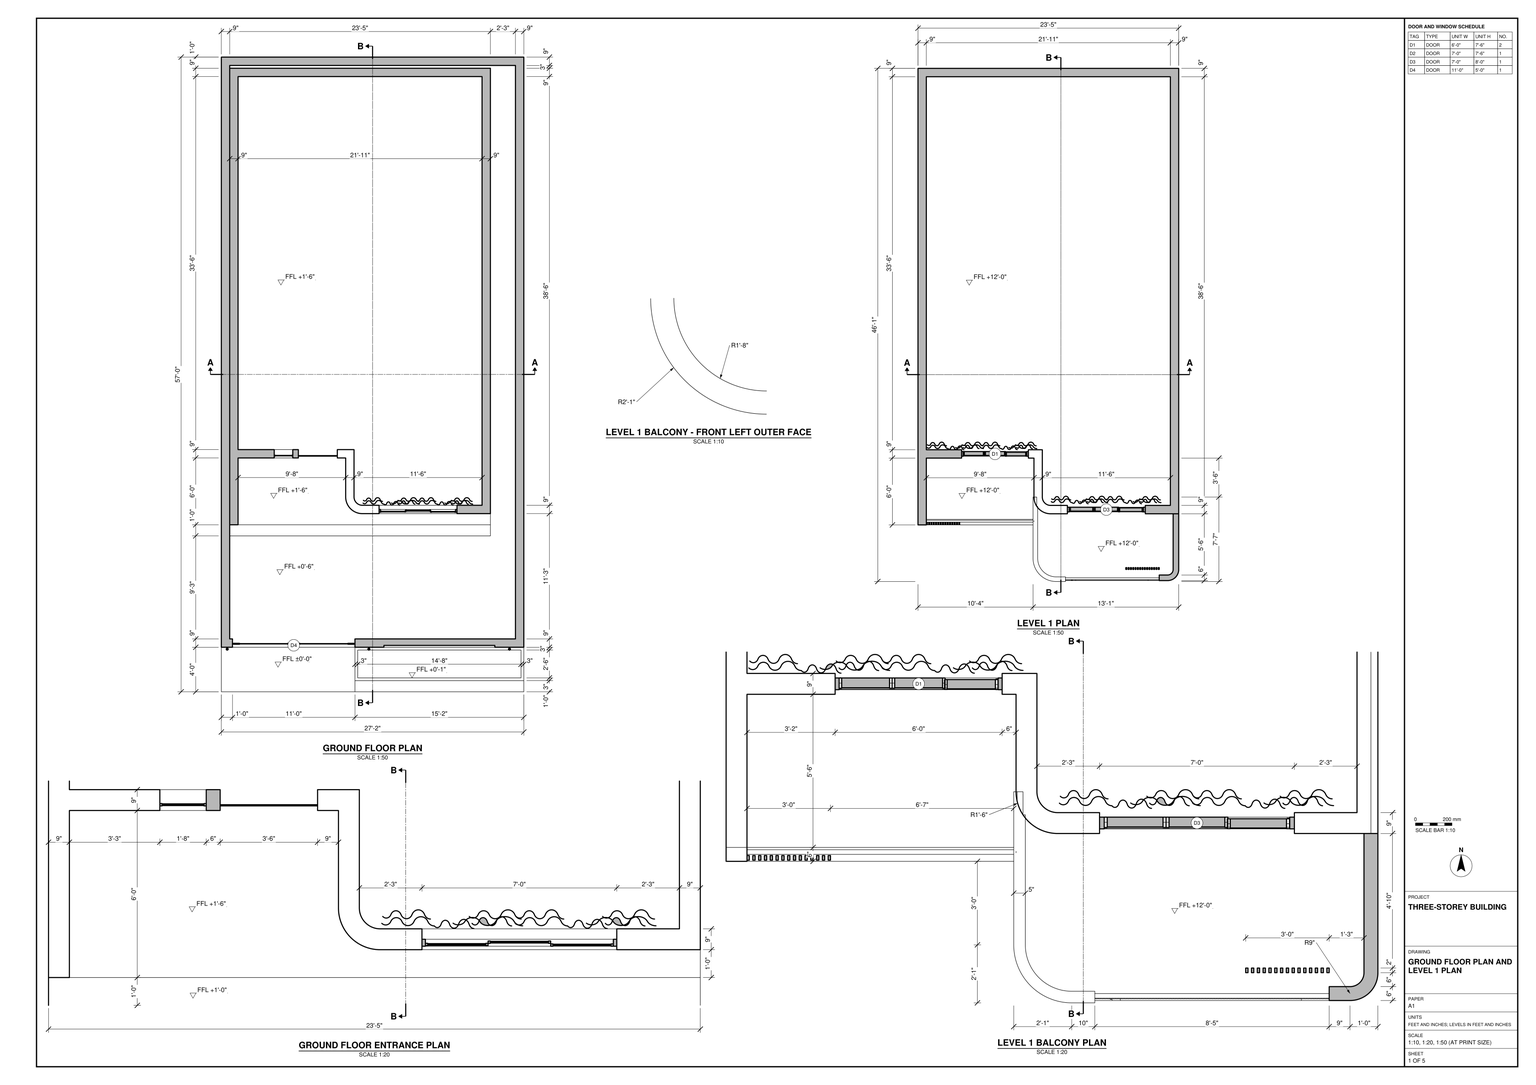
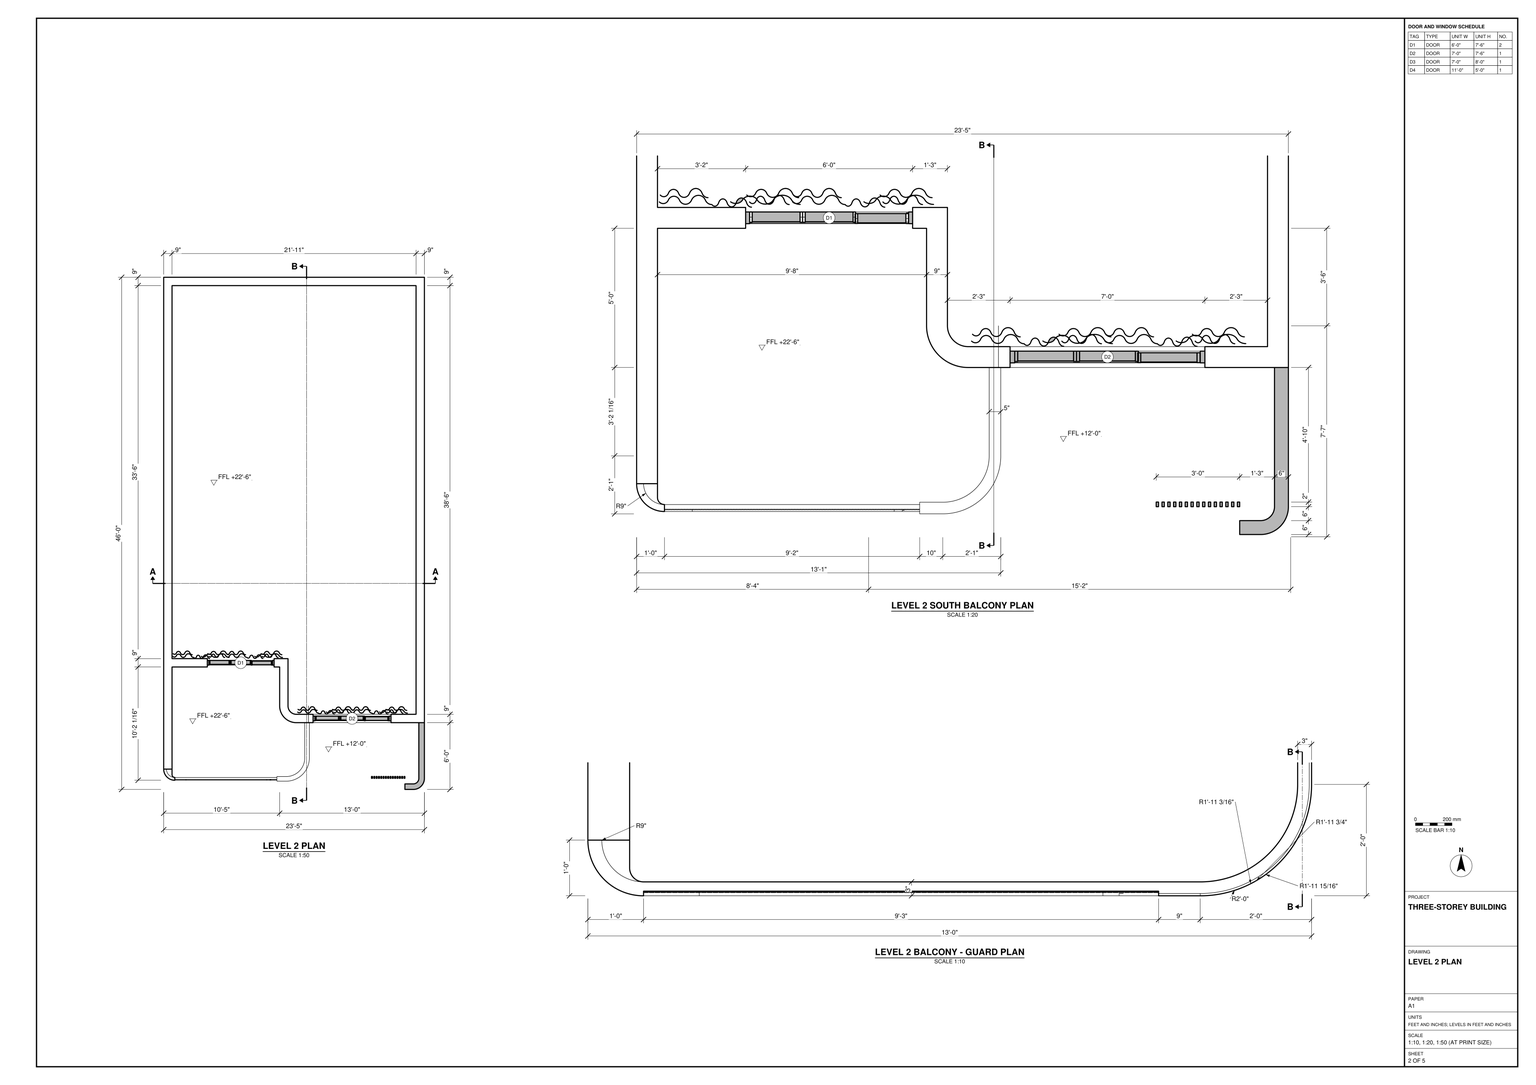
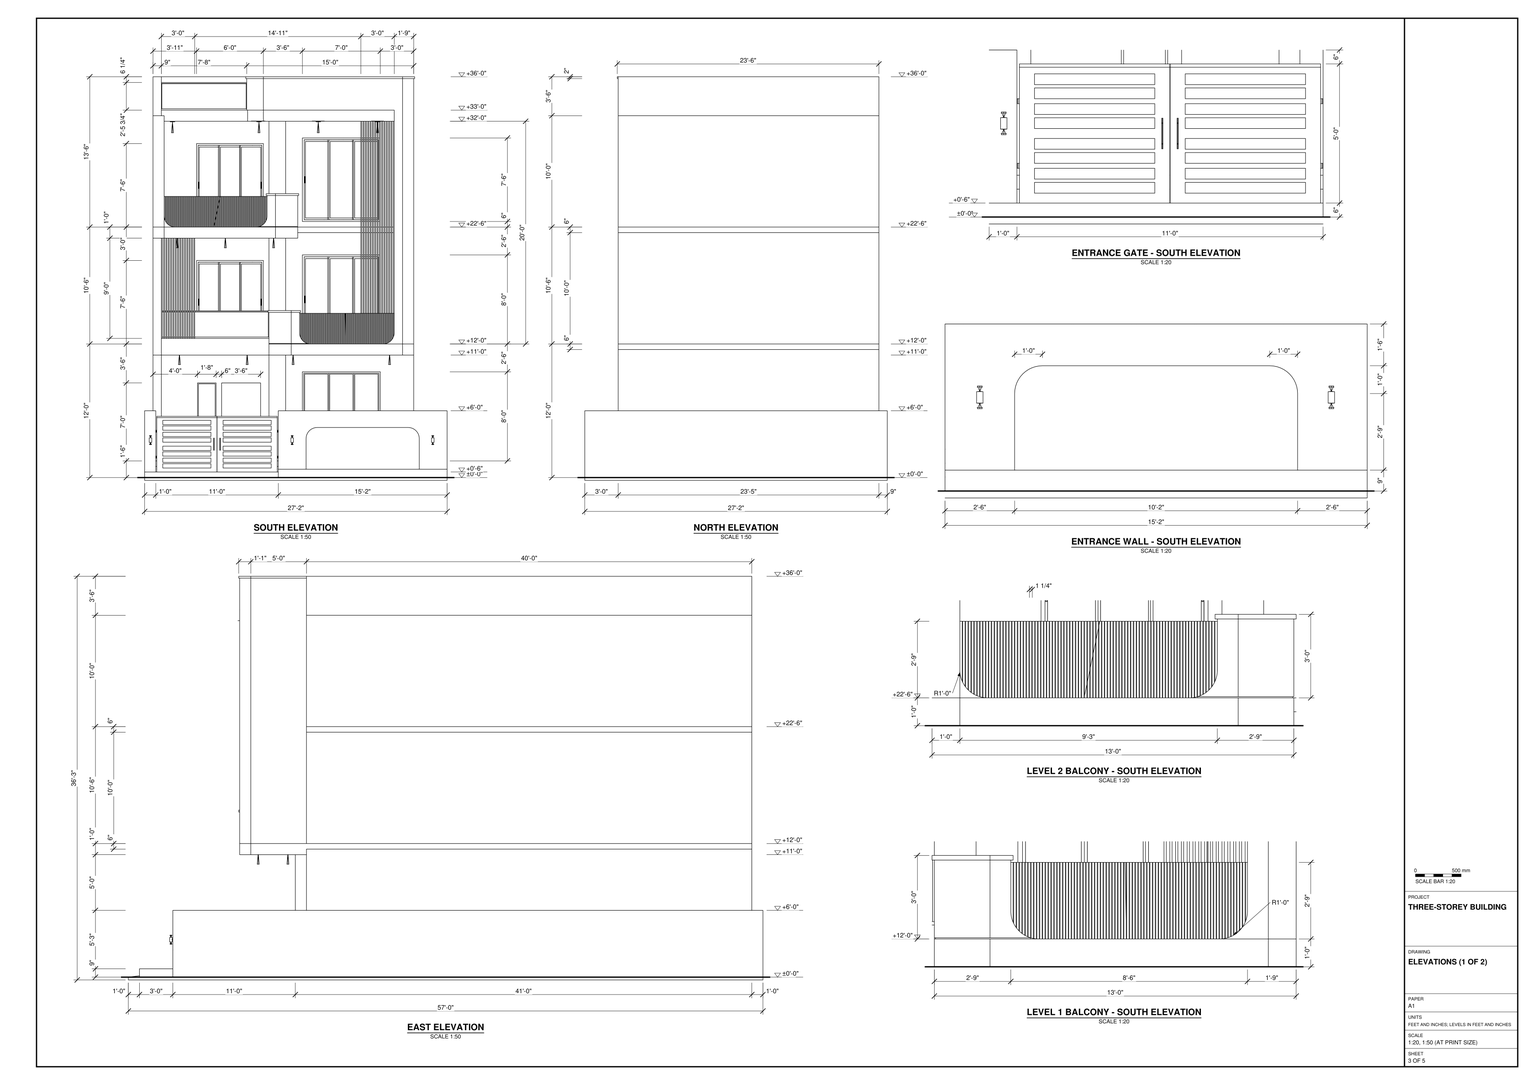
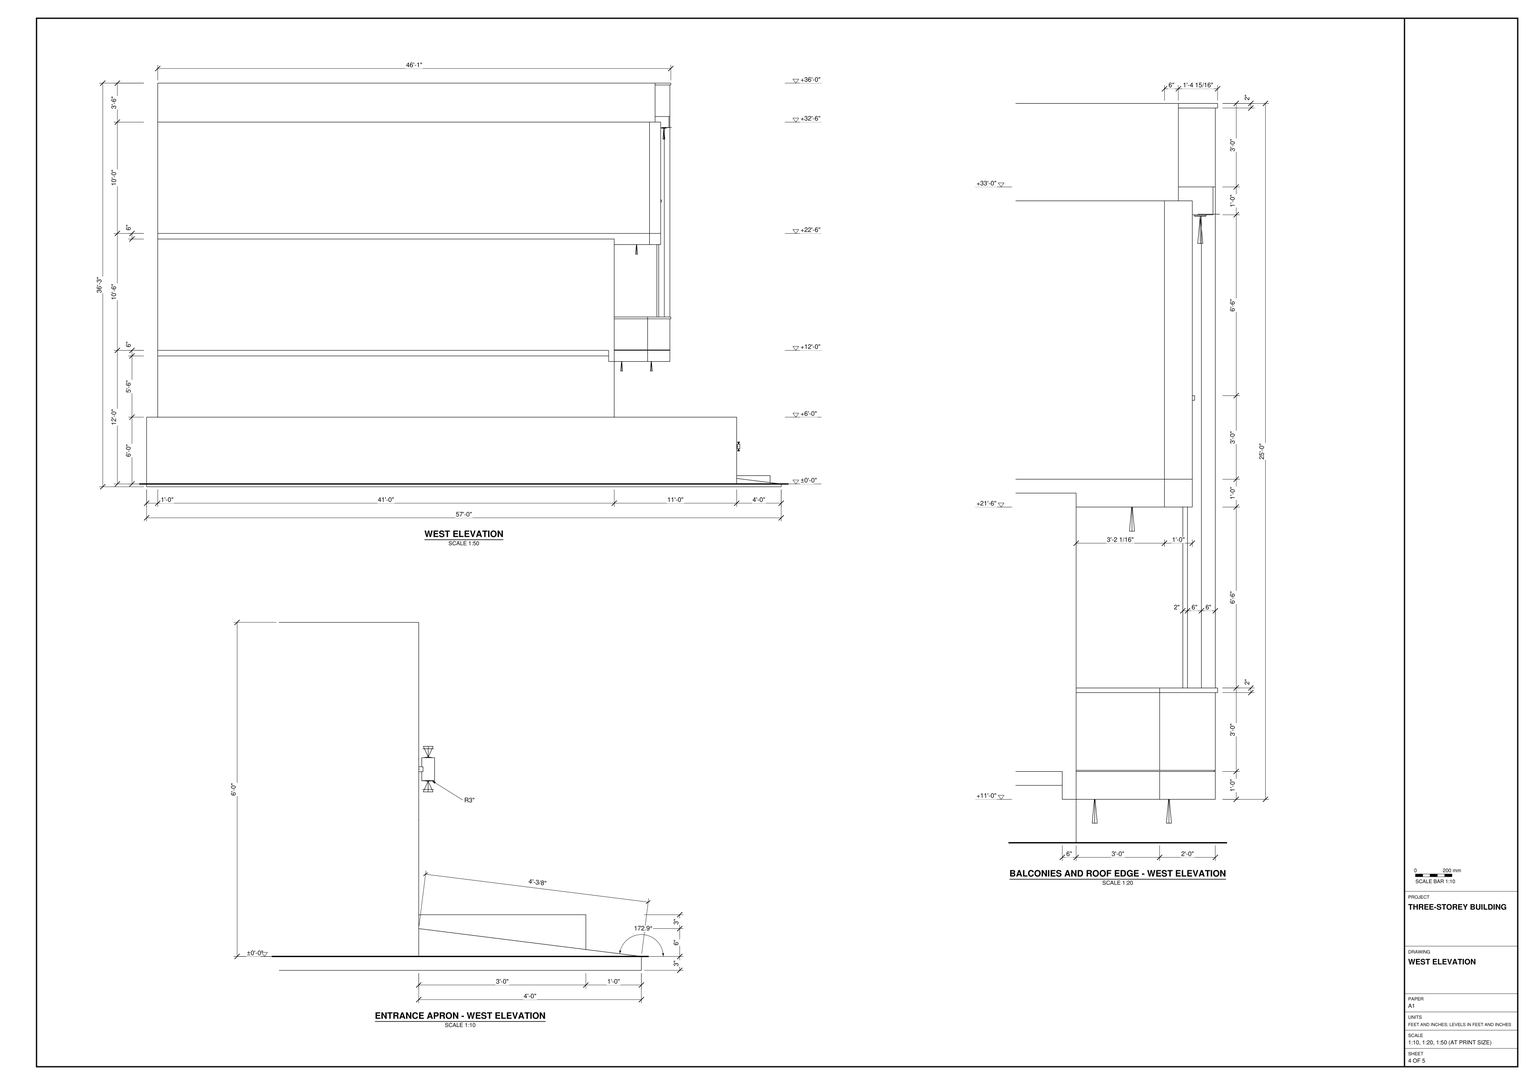
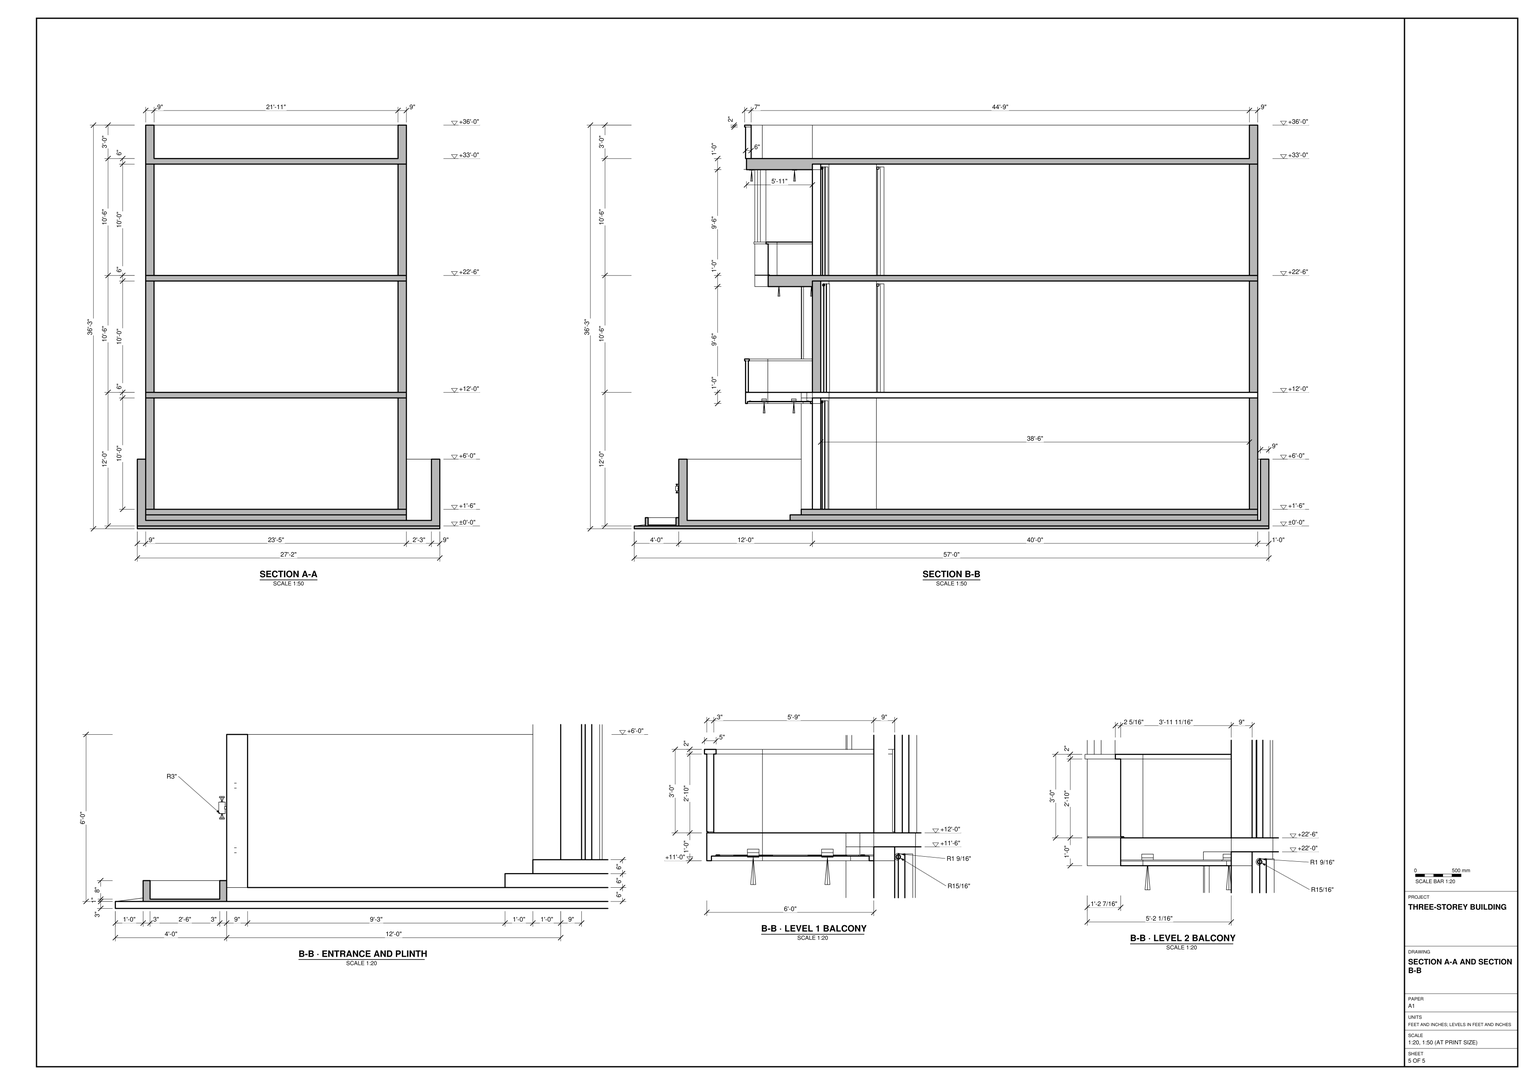
Build the three-storey building and its entrance court in SketchUp from task_files/diagram_01.pdf. Work in feet and inches. Including the court and boundary walls, the model must be 27'-2" wide, 57'-0" deep and 36'-3" high. Use ±0'-0" as the ground datum and set the upper floor levels at +12'-0" and +22'-6".

Start at the south boundary with the double-leaf gate on the left and the entrance wall on the right. Model the changes in height from the court up the shallow steps to the raised ground-floor entrance. Follow the plans for the 9" perimeter walls, the floor slabs and the offset front wall with its curved return. Fit the framed door units into the front openings, keeping the divisions shown in elevation. Leave the main floor areas open as drawn.

Project the level 1 balcony on the right and the level 2 balcony on the left as seen from the south. Use the enlarged details for their slab outlines, curved ends and guards. Distinguish the low balcony guards from the taller vertical screens behind them. Complete the flat roof and its projecting front edge. Keep shell elements such as walls, slabs and roof, and any furniture or joinery pieces, in separate groups or components; use components for repeated parts. Decor and loose items may be any suitable library components. Save one SketchUp model as output_files/three_storey_building_with_staggered_front_balconies.skp.

# SketchUp Ruby script. Lengths in inches.
U = 1.inch
M = Sketchup.active_model
def pt(a) = Geom::Point3d.new(a.map { |v| v * U })
def face(e, loops, mat)
  f = e.add_face(loops[0].map { |a| pt(a) })
  loops[1..].each { |l| e.add_face(l.map { |a| pt(a) }).erase! }
  f.material = f.back_material = mat if mat
  f
end
# faces: each face lists its corners as indices into pts; further lists are holes
def faces(e, pts, list, mat = nil) = list.each { |f| face(e, (f[0].is_a?(Array) ? f : [f]).map { |l| l.map { |i| pts[i] } }, mat) }
# xy, xz, yz: faces in a plane at the given z, y or x. An outline is a flat list of corners, or four numbers for a rectangle; further outlines are holes
def ring(l) = l.size == 4 ? [[l[0], l[1]], [l[2], l[1]], [l[2], l[3]], [l[0], l[3]]] : l.each_slice(2).to_a
def flat(e, list, mat, &to3) = list.each { |f| face(e, (f[0].is_a?(Array) ? f : [f]).map { |l| ring(l).map { |u, v| to3.(u, v) } }, mat) }
def xy(e, z, list, mat = nil) = flat(e, list, mat) { |x, y| [x, y, z] }
def xz(e, y, list, mat = nil) = flat(e, list, mat) { |x, z| [x, y, z] }
def yz(e, x, list, mat = nil) = flat(e, list, mat) { |y, z| [x, y, z] }
def lines(e, pts, list) = list.each { |a, b| e.add_line(pt(pts[a]), pt(pts[b])) }
# prism: a flat outline (further loops are holes) pulled along v
def prism(e, loops, v, mat = nil)
  f = face(e, loops, mat); d = Geom::Vector3d.new(v.map { |x| x * U })
  f.pushpull(f.normal.samedirection?(d) ? d.length : -d.length)
end
def box(e, o, s, mat = nil) = prism(e, [[o, [o[0] + s[0], o[1], o[2]], [o[0] + s[0], o[1] + s[1], o[2]], [o[0], o[1] + s[1], o[2]]]], [0, 0, s[2]], mat)
def at(x, y, z, deg = 0) = Geom::Transformation.translation(pt([x, y, z])) * Geom::Transformation.rotation(ORIGIN, Z_AXIS, deg.degrees)
def axes(o, x, y, z) = Geom::Transformation.new([*x, 0, *y, 0, *z, 0, *pt(o).to_a, 1])
def part(name) = M.definitions.add(name)
# library, detail: a bought-in or finely detailed component or shape, given as its bounding box
def library(name, o, s) = part(name).tap { |d| box(d.entities, o, s) }
def detail(e, o, s) = box(e.add_group.entities, o, s)
def put(e, d, t, mat = nil) = e.add_instance(d, t).tap { |i| i.material = mat if mat }
def group(e, t, mat = nil) = e.add_group.tap { |g| g.transformation = t; g.material = mat if mat }.entities
root = M.entities
M.materials.add("1422 AP 8231 MUTED GREY").color = [95, 93, 94]
M.materials.add("1423 AP 8230 BENTONITE").color = [77, 75, 77]
M.materials.add("1427 AP 686 ARMOUR-N").color = [184, 186, 189]
M.materials.add("[Concrete Block 8x8 Gray]").color = [94, 94, 94]
M.materials.add("[Granite Tile]").color = [155, 148, 143]
M.materials.add("[Granite Tile]1").color = [155, 148, 143]
M.materials.add("[Translucent Glass Blue]").color = [185, 200, 227]
M.materials.add("[Wood Cherry Original]").color = [100, 65, 42]
M.materials.add("[Wood Veneer 01]").color = [99, 65, 43]
c1 = library("Group\#8",[0,-72,0],[281,492,120])
c2 = library("Group\#2",[0,-110.08,0],[281,530.08,120])
c3 = library("Group\#14",[0,-72,-12],[281,492,132])
c4 = library("Group\#13",[-25,-1,0],[182,91,288])
c5 = library("Group\#7",[-9,-81,-16.28],[281,552,58.03])
c6 = library("Group\#12",[-9,-71.08,-16.4],[281,542.08,22.4])
c7 = library("Group\#9",[-1,-1,0],[157,81.05,120])
c8 = part("Group188\#1")
box(c8.entities,[-18,-57,0],[1,114,2])
c9 = part("Group189\#1")
box(c9.entities,[-15.5,-57,0],[1,114,2])
c10 = part("Group190\#1")
box(c10.entities,[-13,-57,0],[1,114,2])
c11 = part("Group191\#1")
box(c11.entities,[-10.5,-57,0],[1,114,2])
c12 = part("Group192\#1")
box(c12.entities,[-8,-57,0],[1,114,2])
c13 = part("Group193\#1")
box(c13.entities,[-5.5,-57,0],[1,114,2])
c14 = part("Group194\#1")
box(c14.entities,[-3,-57,0],[1,114,2])
c15 = part("Group195\#1")
box(c15.entities,[-0.5,-57,0],[1,114,2])
c16 = part("Group196\#1")
box(c16.entities,[2,-57,0],[1,114,2])
c17 = part("Group197\#1")
box(c17.entities,[4.5,-57,0],[1,114,2])
c18 = part("Group198\#1")
box(c18.entities,[7,-57,0],[1,114,2])
c19 = part("Group199\#1")
box(c19.entities,[9.5,-57,0],[1,114,2])
c20 = part("Group200\#1")
box(c20.entities,[12,-57,0],[1,114,2])
c21 = part("Group201\#1")
box(c21.entities,[14.5,-57,0],[1,114,2])
c22 = part("Group202\#1")
box(c22.entities,[17,-57,0],[1,114,2])
c23 = part("Group186\#1")
put(c23.entities,c8,at(0,0,0))
put(c23.entities,c9,at(0,0,0))
put(c23.entities,c10,at(0,0,0))
put(c23.entities,c11,at(0,0,0))
put(c23.entities,c12,at(0,0,0))
put(c23.entities,c13,at(0,0,0))
put(c23.entities,c14,at(0,0,0))
put(c23.entities,c15,at(0,0,0))
put(c23.entities,c16,at(0,0,0))
put(c23.entities,c17,at(0,0,0))
put(c23.entities,c18,at(0,0,0))
put(c23.entities,c19,at(0,0,0))
put(c23.entities,c20,at(0,0,0))
put(c23.entities,c21,at(0,0,0))
put(c23.entities,c22,at(0,0,0))
c24 = part("Group\#19")
put(c24.entities,c23,axes([18,0,57],[1,0,0],[0,0,1],[0,-1,0]))
c25 = library("Group\#15",[-9,-82.92,-18.4],[281,553.92,60.4])
c26 = library("Gate",[-1,-3.25,0],[122,4.25,84])
c27 = library("WALL LIGHT 69\#1",[4.19,4.05,-8.39],[4.61,5.7,16.35])
g1 = group(root,at(9,252,0))
g2 = group(g1,at(0,-133,-12))
box(g2,[9,37.5,378],[93,11,12],"1423 AP 8230 BENTONITE")
put(g2,c1,at(0,133,12),"1427 AP 686 ARMOUR-N")
put(g2,c2,at(0,133,264),"1427 AP 686 ARMOUR-N")
put(g2,c3,at(0,133,138),"1423 AP 8230 BENTONITE")
g3 = group(g2,at(0,73,6),"[Granite Tile]")
box(g3,[0,-24,-6],[281,504,6])
g4 = group(g2,at(0,73,12),"[Granite Tile]")
box(g4,[0,-12,-6],[281,492,6])
put(g2,c4,at(125,1,138),"1427 AP 686 ARMOUR-N")
put(g2,c5,at(9,82,132))
put(g2,c6,at(9,82,258))
put(g2,c7,axes([156,10.92,264],[-1,0,0],[0,1,0],[0,0,1]),"1427 AP 686 ARMOUR-N")
put(g2,c24,axes([9,63.5,144],[1,0,0],[0,1,0],[0,0,0.94737]),"[Wood Cherry Original]")
put(g2,c24,axes([224,15,138],[1,0,0],[0,1,0],[0,0,2.10526]),"[Wood Cherry Original]")
put(g2,c25,at(9,82,384))
g5 = group(g2,at(37.55,69,390),"[Wood Veneer 01]")
xy(g5,0,[[-28.55,0,63.45,2]])
xy(g5,1.25,[[-27.96,0.75,62.85,1.25]])
xy(g5,1.5,[[[-28.55,0,63.45,2],[-27.96,0.75,62.85,1.25]]])
xy(g5,28.5,[[-28.55,0.2,63.45,0.23],[-28.55,0.23,63.45,0.25],[[-28.55,0.25,63.45,1.75],[-27.96,0.75,62.85,1.25]],[-28.55,1.75,63.45,1.77],[-28.55,1.77,63.45,1.8]])
xy(g5,28.75,[[-27.96,0.75,62.85,1.25]])
xy(g5,29.74,[[-28.55,0.84,63.45,0.9],[-28.55,1.1,63.45,1.16]])
xy(g5,29.75,[[-28.55,0.95,63.45,1],[-28.55,1,63.45,1.05]])
xz(g5,0,[[-28.55,0,63.45,1.5],[-28.55,28.7,63.45,28.73],[-28.55,28.73,63.45,28.75],[-28.55,28.75,63.45,28.8]])
xz(g5,0.01,[[-28.55,28.85,63.45,28.91]])
xz(g5,0.75,[[-27.96,1.25,62.85,1.5],[-27.96,28.5,62.85,28.75]])
xz(g5,1.25,[[-27.96,1.25,62.85,1.5],[-27.96,28.5,62.85,28.75]])
xz(g5,1.99,[[-28.55,28.85,63.45,28.91]])
xz(g5,2,[[-28.55,0,63.45,1.5],[-28.55,28.7,63.45,28.73],[-28.55,28.73,63.45,28.75],[-28.55,28.75,63.45,28.8]])
yz(g5,-28.55,[[0,0,2,1.5],[0.2,28.5,0.18,28.51,0.15,28.52,0.11,28.54,0.09,28.56,0.07,28.57,0.06,28.59,0.04,28.61,0.02,28.65,0.01,28.68,0,28.7,0,28.8,0.01,28.85,0.01,28.91,0.03,29.01,0.09,29.16,0.11,29.2,0.13,29.25,0.16,29.29,0.19,29.34,0.22,29.38,0.26,29.42,0.29,29.46,0.33,29.49,0.37,29.53,0.41,29.56,0.46,29.59,0.5,29.62,0.55,29.64,0.59,29.66,0.74,29.72,0.84,29.74,0.9,29.74,0.95,29.75,1.05,29.75,1.1,29.74,1.16,29.74,1.26,29.72,1.41,29.66,1.45,29.64,1.5,29.62,1.54,29.59,1.59,29.56,1.63,29.53,1.67,29.49,1.71,29.46,1.74,29.42,1.78,29.38,1.81,29.34,1.84,29.29,1.87,29.25,1.89,29.2,1.91,29.16,1.97,29.01,1.99,28.91,1.99,28.85,2,28.8,2,28.7,1.99,28.68,1.98,28.65,1.96,28.61,1.94,28.59,1.93,28.57,1.91,28.56,1.89,28.54,1.85,28.52,1.82,28.51,1.8,28.5]])
yz(g5,-27.96,[[0.75,1.25,1.25,1.5],[0.75,28.5,1.25,28.75]])
yz(g5,62.85,[[0.75,1.25,1.25,1.5],[0.75,28.5,1.25,28.75]])
yz(g5,63.45,[[0,0,2,1.5],[0.2,28.5,1.8,28.5,1.82,28.51,1.85,28.52,1.89,28.54,1.91,28.56,1.93,28.57,1.94,28.59,1.96,28.61,1.98,28.65,1.99,28.68,2,28.7,2,28.8,1.99,28.85,1.99,28.91,1.97,29.01,1.91,29.16,1.89,29.2,1.87,29.25,1.84,29.29,1.81,29.34,1.78,29.38,1.74,29.42,1.71,29.46,1.67,29.49,1.63,29.53,1.59,29.56,1.54,29.59,1.5,29.62,1.45,29.64,1.41,29.66,1.26,29.72,1.16,29.74,1.1,29.74,1.05,29.75,0.95,29.75,0.9,29.74,0.84,29.74,0.74,29.72,0.59,29.66,0.55,29.64,0.5,29.62,0.46,29.59,0.41,29.56,0.37,29.53,0.33,29.49,0.29,29.46,0.26,29.42,0.22,29.38,0.19,29.34,0.16,29.29,0.13,29.25,0.11,29.2,0.09,29.16,0.03,29.01,0.01,28.91,0.01,28.85,0,28.8,0,28.7,0.01,28.68,0.02,28.65,0.04,28.61,0.06,28.59,0.07,28.57,0.09,28.56,0.11,28.54,0.15,28.52,0.18,28.51]])
p = [[-28.55,0.13,28.53],[-28.55,0.15,28.52],[63.45,0.15,28.52],[63.45,0.13,28.53],[-28.55,0.11,28.54],[63.45,0.11,28.54],
  [-28.55,0.09,28.56],[63.45,0.09,28.56],[-28.55,0.18,28.51],[-28.55,0.2,28.5],[63.45,0.2,28.5],[63.45,0.18,28.51],
  [-28.55,1.85,28.52],[-28.55,1.87,28.53],[63.45,1.87,28.53],[63.45,1.85,28.52],[-28.55,1.82,28.51],[63.45,1.82,28.51],
  [-28.55,1.8,28.5],[63.45,1.8,28.5],[-28.55,1.89,28.54],[-28.55,1.91,28.56],[63.45,1.91,28.56],[63.45,1.89,28.54],
  [-28.55,0.04,28.61],[-28.55,0.06,28.59],[63.45,0.06,28.59],[63.45,0.04,28.61],[-28.55,0.03,28.63],[63.45,0.03,28.63],
  [-28.55,0.02,28.65],[63.45,0.02,28.65],[-28.55,0.07,28.57],[63.45,0.07,28.57],[-28.55,1.94,28.59],[-28.55,1.96,28.61],
  [63.45,1.96,28.61],[63.45,1.94,28.59],[-28.55,1.93,28.57],[63.45,1.93,28.57],[-28.55,1.97,28.63],[-28.55,1.98,28.65],
  [63.45,1.98,28.65],[63.45,1.97,28.63],[-28.55,0.01,28.68],[63.45,0.01,28.68],[-28.55,0,28.7],[63.45,0,28.7],
  [-28.55,1.99,28.68],[-28.55,2,28.7],[63.45,2,28.7],[63.45,1.99,28.68],[-28.55,0.01,28.85],[-28.55,0,28.8],
  [63.45,0,28.8],[63.45,0.01,28.85],[-28.55,2,28.8],[-28.55,1.99,28.85],[63.45,1.99,28.85],[63.45,2,28.8],
  [-28.55,0.02,28.96],[-28.55,0.01,28.91],[63.45,0.01,28.91],[63.45,0.02,28.96],[-28.55,1.99,28.91],[-28.55,1.98,28.96],
  [63.45,1.98,28.96],[63.45,1.99,28.91],[-28.55,0.03,29.01],[63.45,0.03,29.01],[-28.55,0.05,29.06],[63.45,0.05,29.06],
  [-28.55,1.97,29.01],[-28.55,1.95,29.06],[63.45,1.95,29.06],[63.45,1.97,29.01],[-28.55,0.07,29.11],[63.45,0.07,29.11],
  [-28.55,0.09,29.16],[63.45,0.09,29.16],[-28.55,1.93,29.11],[-28.55,1.91,29.16],[63.45,1.91,29.16],[63.45,1.93,29.11],
  [-28.55,0.11,29.2],[63.45,0.11,29.2],[-28.55,0.13,29.25],[63.45,0.13,29.25],[-28.55,1.89,29.2],[-28.55,1.87,29.25],
  [63.45,1.87,29.25],[63.45,1.89,29.2],[-28.55,0.16,29.29],[63.45,0.16,29.29],[-28.55,0.19,29.34],[63.45,0.19,29.34],
  [-28.55,0.22,29.38],[63.45,0.22,29.38],[-28.55,1.81,29.34],[-28.55,1.78,29.38],[63.45,1.78,29.38],[63.45,1.81,29.34],
  [-28.55,1.84,29.29],[63.45,1.84,29.29],[-28.55,0.26,29.42],[63.45,0.26,29.42],[-28.55,0.29,29.46],[63.45,0.29,29.46],
  [-28.55,1.74,29.42],[-28.55,1.71,29.46],[63.45,1.71,29.46],[63.45,1.74,29.42],[-28.55,0.33,29.49],[63.45,0.33,29.49],
  [-28.55,0.37,29.53],[63.45,0.37,29.53],[-28.55,0.41,29.56],[63.45,0.41,29.56],[-28.55,1.63,29.53],[-28.55,1.59,29.56],
  [63.45,1.59,29.56],[63.45,1.63,29.53],[-28.55,1.67,29.49],[63.45,1.67,29.49],[-28.55,0.46,29.59],[63.45,0.46,29.59],
  [-28.55,0.5,29.62],[63.45,0.5,29.62],[-28.55,0.55,29.64],[63.45,0.55,29.64],[-28.55,0.59,29.66],[63.45,0.59,29.66],
  [-28.55,1.45,29.64],[-28.55,1.41,29.66],[63.45,1.41,29.66],[63.45,1.45,29.64],[-28.55,1.5,29.62],[63.45,1.5,29.62],
  [-28.55,1.54,29.59],[63.45,1.54,29.59],[-28.55,0.64,29.68],[63.45,0.64,29.68],[-28.55,0.69,29.7],[63.45,0.69,29.7],
  [-28.55,0.74,29.72],[63.45,0.74,29.72],[-28.55,0.79,29.73],[63.45,0.79,29.73],[-28.55,0.84,29.74],[63.45,0.84,29.74],
  [-28.55,0.95,29.75],[-28.55,0.9,29.74],[63.45,0.9,29.74],[63.45,0.95,29.75],[-28.55,1.1,29.74],[-28.55,1.05,29.75],
  [63.45,1.05,29.75],[63.45,1.1,29.74],[-28.55,1.21,29.73],[-28.55,1.16,29.74],[63.45,1.16,29.74],[63.45,1.21,29.73],
  [-28.55,1.26,29.72],[63.45,1.26,29.72],[-28.55,1.31,29.7],[63.45,1.31,29.7],[-28.55,1.36,29.68],[63.45,1.36,29.68]]
faces(g5,p,[[0,1,2,3],[4,0,3,5],[6,4,5,7],[8,9,10,11],[1,8,11,2],[12,13,14,15],[16,12,15,17],[18,16,17,19],
  [20,21,22,23],[13,20,23,14],[24,25,26,27],[28,24,27,29],[30,28,29,31],[32,6,7,33],[25,32,33,26],[34,35,36,37],
  [38,34,37,39],[21,38,39,22],[40,41,42,43],[35,40,43,36],[44,30,31,45],[46,44,45,47],[48,49,50,51],[41,48,51,42],
  [52,53,54,55],[56,57,58,59],[60,61,62,63],[64,65,66,67],[68,60,63,69],[70,68,69,71],[72,73,74,75],[65,72,75,66],
  [76,70,71,77],[78,76,77,79],[80,81,82,83],[73,80,83,74],[84,78,79,85],[86,84,85,87],[88,89,90,91],[81,88,91,82],
  [92,86,87,93],[94,92,93,95],[96,94,95,97],[98,99,100,101],[102,98,101,103],[89,102,103,90],[104,96,97,105],[106,104,105,107],
  [108,109,110,111],[99,108,111,100],[112,106,107,113],[114,112,113,115],[116,114,115,117],[118,119,120,121],[122,118,121,123],[109,122,123,110],
  [124,116,117,125],[126,124,125,127],[128,126,127,129],[130,128,129,131],[132,133,134,135],[136,132,135,137],[138,136,137,139],[119,138,139,120],
  [140,130,131,141],[142,140,141,143],[144,142,143,145],[146,144,145,147],[148,146,147,149],[150,151,152,153],[154,155,156,157],[158,159,160,161],
  [162,158,161,163],[164,162,163,165],[166,164,165,167],[133,166,167,134]])
g6 = group(g5,at(0.59,0.75,1.25),"[Translucent Glass Blue]")
box(g6,[-28.55,0,0],[90.81,0.5,27.5])
g7 = group(g2,at(0,49,0),"1427 AP 686 ARMOUR-N")
xy(g7,-6,[[-9,-120,-9,516,317,516,317,-120,287,-120,287,-118,165,-118,165,-120],[165,-120,287,-118]])
xy(g7,0,[[3,-120,135,-120,135,-111,308,-111,308,507,0,507,0,-111,3,-111]],"[Granite Tile]")
xy(g7,48,[[177,-120,275,-118]])
xy(g7,66,[[-9,-120,3,-120,3,-111,0,-111,0,507,308,507,308,-111,135,-111,135,-120,317,-120,317,516,-9,516]])
xz(g7,-120,[[-9,-6,165,-6,165,36,165.1,37.57,165.41,39.11,165.91,40.59,166.61,42,167.48,43.31,168.51,44.49,169.69,45.52,171,46.39,172.41,47.09,173.89,47.59,175.43,47.9,177,48,275,48,276.57,47.9,278.11,47.59,279.59,47.09,281,46.39,282.31,45.52,283.49,44.49,284.52,43.31,285.39,42,286.09,40.59,286.59,39.11,286.9,37.57,287,36,287,-6,317,-6,317,66,135,66,135,0,3,0,3,66,-9,66]])
xz(g7,-118,[[165,-6,287,-6,287,36,286.9,37.57,286.59,39.11,286.09,40.59,285.39,42,284.52,43.31,283.49,44.49,282.31,45.52,281,46.39,279.59,47.09,278.11,47.59,276.57,47.9,275,48,177,48,175.43,47.9,173.89,47.59,172.41,47.09,171,46.39,169.69,45.52,168.51,44.49,167.48,43.31,166.61,42,165.91,40.59,165.41,39.11,165.1,37.57,165,36]],"1422 AP 8231 MUTED GREY")
xz(g7,-111,[[0,0,3,66],[135,0,308,66]])
xz(g7,507,[[0,0,308,66]])
xz(g7,516,[[-9,-6,317,66]])
yz(g7,-9,[[-120,-6,516,66]])
yz(g7,0,[[-111,0,507,66]])
yz(g7,3,[[-120,0,-111,66]])
yz(g7,135,[[-120,0,-111,66]])
yz(g7,165,[[-120,-6,-118,36]])
yz(g7,287,[[-120,-6,-118,36]])
yz(g7,308,[[-111,0,507,66]])
yz(g7,317,[[-120,-6,516,66]])
p = [[165.1,-120,37.57],[165,-120,36],[165,-118,36],[165.1,-118,37.57],[287,-120,36],[286.9,-120,37.57],
  [286.9,-118,37.57],[287,-118,36],[165.41,-120,39.11],[165.41,-118,39.11],[286.59,-120,39.11],[286.59,-118,39.11],
  [165.91,-120,40.59],[165.91,-118,40.59],[286.09,-120,40.59],[286.09,-118,40.59],[166.61,-120,42],[166.61,-118,42],
  [285.39,-120,42],[285.39,-118,42],[167.48,-120,43.31],[167.48,-118,43.31],[284.52,-120,43.31],[284.52,-118,43.31],
  [168.51,-120,44.49],[168.51,-118,44.49],[283.49,-120,44.49],[283.49,-118,44.49],[169.69,-120,45.52],[169.69,-118,45.52],
  [282.31,-120,45.52],[282.31,-118,45.52],[171,-120,46.39],[171,-118,46.39],[281,-120,46.39],[281,-118,46.39],
  [172.41,-120,47.09],[172.41,-118,47.09],[279.59,-120,47.09],[279.59,-118,47.09],[173.89,-120,47.59],[173.89,-118,47.59],
  [278.11,-120,47.59],[278.11,-118,47.59],[175.43,-120,47.9],[175.43,-118,47.9],[276.57,-120,47.9],[276.57,-118,47.9],
  [177,-120,48],[177,-118,48],[275,-120,48],[275,-118,48]]
faces(g7,p,[[0,1,2,3],[4,5,6,7],[8,0,3,9],[5,10,11,6],[12,8,9,13],[10,14,15,11],[16,12,13,17],[14,18,19,15],
  [20,16,17,21],[18,22,23,19],[24,20,21,25],[22,26,27,23],[28,24,25,29],[26,30,31,27],[32,28,29,33],[30,34,35,31],
  [36,32,33,37],[34,38,39,35],[40,36,37,41],[38,42,43,39],[44,40,41,45],[42,46,47,43],[48,44,45,49],[46,50,51,47]])
put(g7,c26,axes([4.08,-116.75,0],[1.08197,0,0],[0,1,0],[0,0,0.71429]))
put(g7,c27,axes([146.1,-125.85,34.51],[0.6,0,0],[0,0.6,0],[0,0,0.6]))
put(g7,c27,axes([297.66,-125.85,34.51],[0.6,0,0],[0,0.6,0],[0,0,0.6]))
put(g7,c27,axes([-6.58,-125.85,34.51],[0.6,0,0],[0,0.6,0],[0,0,0.6]))
g8 = group(g7,at(135,-137.27,-6),"[Concrete Block 8x8 Gray]")
xy(g8,0,[[0,-18.75,182,17.27]])
xy(g8,1,[[3,-15.75,179,14.27]])
xy(g8,9,[[[0,-18.75,182,17.27],[3,-15.75,179,14.27]]])
xz(g8,-18.75,[[0,0,182,9]])
xz(g8,-15.75,[[3,1,179,9]])
xz(g8,14.27,[[3,1,179,9]])
xz(g8,17.27,[[0,0,30,9],[30,0,152,9],[152,0,182,9]])
yz(g8,0,[[-18.75,0,17.27,9]])
yz(g8,3,[[-15.75,1,14.27,9]])
yz(g8,179,[[-15.75,1,14.27,9]])
yz(g8,182,[[-18.75,0,17.27,9]])
g9 = group(g2,at(2.89,-71,-6))
xy(g9,0,[[-11.89,-48,132.11,0]])
xz(g9,0,[[-11.89,0,132.11,6]])
yz(g9,-11.89,[[-48,0,0,6,0,0]])
yz(g9,132.11,[[-48,0,0,0,0,6]])
p = [[132.11,0,6],[-11.89,0,6],[-11.89,-48,0],[132.11,-48,0]]
faces(g9,p,[[0,1,2,3]],"[Granite Tile]1")
g10 = group(g2,at(-9,-107.02,-6))
box(g10,[0,-11.98,-3],[326,684,3])
